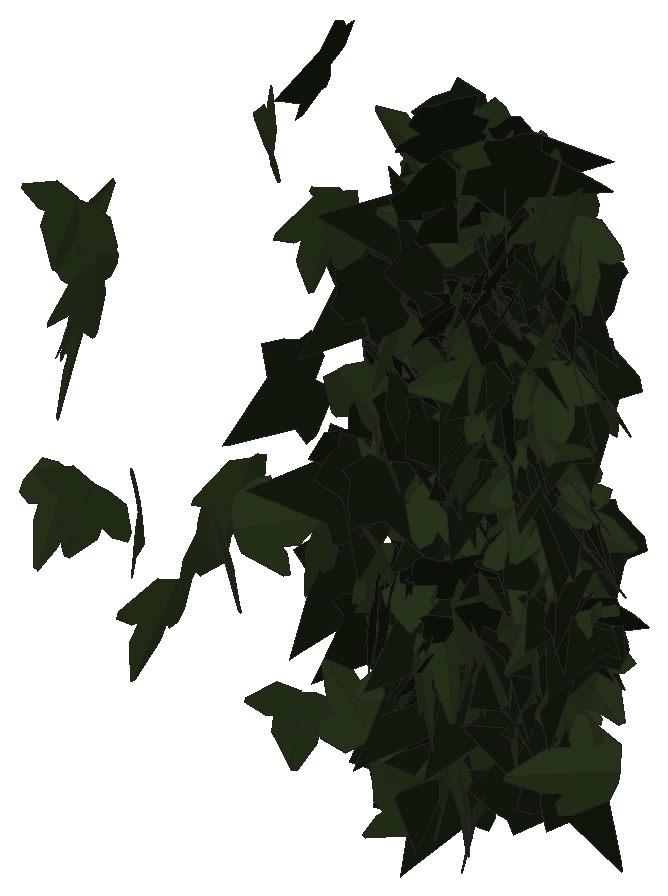
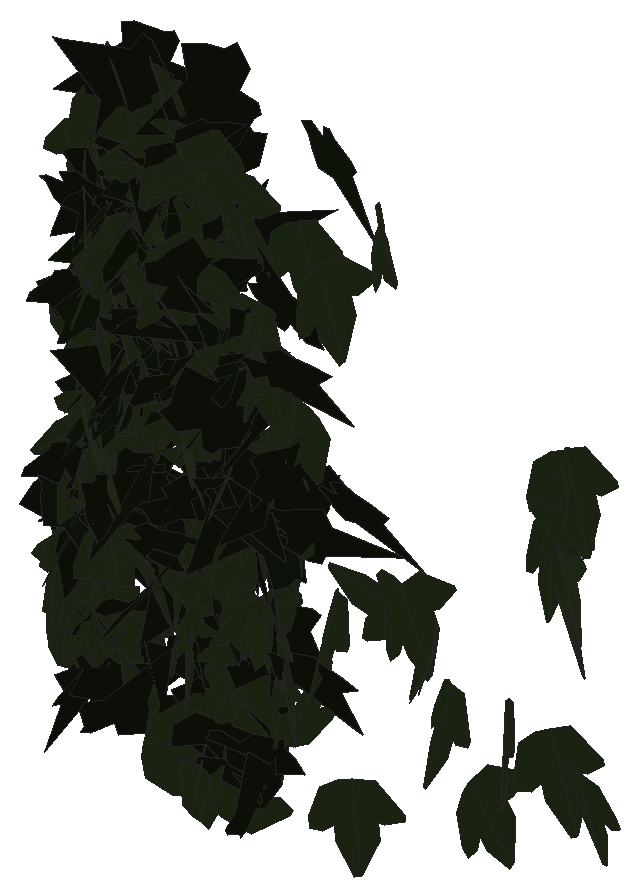
# SketchUp Ruby script. Lengths in inches.
U = 1.inch
M = Sketchup.active_model
def pt(a) = Geom::Point3d.new(a.map { |v| v * U })
def face(e, loops, mat)
  f = e.add_face(loops[0].map { |a| pt(a) })
  loops[1..].each { |l| e.add_face(l.map { |a| pt(a) }).erase! }
  f.material = f.back_material = mat if mat
  f
end
# faces: each face lists its corners as indices into pts; further lists are holes
def faces(e, pts, list, mat = nil) = list.each { |f| face(e, (f[0].is_a?(Array) ? f : [f]).map { |l| l.map { |i| pts[i] } }, mat) }
# xy, xz, yz: faces in a plane at the given z, y or x. An outline is a flat list of corners, or four numbers for a rectangle; further outlines are holes
def ring(l) = l.size == 4 ? [[l[0], l[1]], [l[2], l[1]], [l[2], l[3]], [l[0], l[3]]] : l.each_slice(2).to_a
def flat(e, list, mat, &to3) = list.each { |f| face(e, (f[0].is_a?(Array) ? f : [f]).map { |l| ring(l).map { |u, v| to3.(u, v) } }, mat) }
def xy(e, z, list, mat = nil) = flat(e, list, mat) { |x, y| [x, y, z] }
def xz(e, y, list, mat = nil) = flat(e, list, mat) { |x, z| [x, y, z] }
def yz(e, x, list, mat = nil) = flat(e, list, mat) { |y, z| [x, y, z] }
def lines(e, pts, list) = list.each { |a, b| e.add_line(pt(pts[a]), pt(pts[b])) }
# prism: a flat outline (further loops are holes) pulled along v
def prism(e, loops, v, mat = nil)
  f = face(e, loops, mat); d = Geom::Vector3d.new(v.map { |x| x * U })
  f.pushpull(f.normal.samedirection?(d) ? d.length : -d.length)
end
def box(e, o, s, mat = nil) = prism(e, [[o, [o[0] + s[0], o[1], o[2]], [o[0] + s[0], o[1] + s[1], o[2]], [o[0], o[1] + s[1], o[2]]]], [0, 0, s[2]], mat)
def at(x, y, z, deg = 0) = Geom::Transformation.translation(pt([x, y, z])) * Geom::Transformation.rotation(ORIGIN, Z_AXIS, deg.degrees)
def axes(o, x, y, z) = Geom::Transformation.new([*x, 0, *y, 0, *z, 0, *pt(o).to_a, 1])
def part(name) = M.definitions.add(name)
# library, detail: a bought-in or finely detailed component or shape, given as its bounding box
def library(name, o, s) = part(name).tap { |d| box(d.entities, o, s) }
def detail(e, o, s) = box(e.add_group.entities, o, s)
def put(e, d, t, mat = nil) = e.add_instance(d, t).tap { |i| i.material = mat if mat }
def group(e, t, mat = nil) = e.add_group.tap { |g| g.transformation = t; g.material = mat if mat }.entities
root = M.entities
M.materials.add("efeu1").color = [18, 25, 13]
M.materials.add("efeu2").color = [43, 57, 29]
c1 = part("ivyleaf_9")
p = [[1.54,2.16,1.25],[1.36,2.04,1.19],[-0.21,0.99,0.68],[-0.71,1.11,0.82],[-0.85,0.86,0.67],[-0.8,0.17,0.21],
  [-0.9,-0.01,0.1],[-0.67,-0.16,-0.02],[-0.08,-0.08,-0.05],[-0.03,-0.6,-0.4],[0.65,-0.88,-0.66],[0.83,-0.6,-0.49],
  [1.29,-0.42,-0.43],[1.8125,-0.07,-0.26],[1.21,0.44,0.15]]
faces(c1.entities,p,[[0,1,2,3,4,5,6,7,8,9,10,11,12,13,14]],"efeu1")
c2 = part("ivyleaf_10")
p = [[0,0.5,-0.03],[-0.0625,2.02,-0.43],[-0.19,2.01,-0.46],[-0.54,1.05,-0.29],[-0.52,0.625,-0.18],[-0.83,0.76,-0.28],
  [-1.16,0.64,-0.33],[-1.15,0.33,-0.24],[-0.77,-0.39,0.02],[-0.3,-0.51,0.16],[0.04,-0.48,0.23],[-0.02,2.01,-0.4375],
  [-0.06,2.01,-0.43],[0.04,-0.49,0.23],[0.67,-0.49,0.14],[1.38,0.36,-0.2],[1.375,0.51,-0.24],[0.81,0.65,-0.19],
  [0.62,0.59,-0.15],[0.6,1.09,-0.28],[0.5,1.23,-0.31]]
faces(c2.entities,p,[[0,1,2,3,4,5,6,7,8,9,10],[11,12,0,13,14,15,16,17,18,19,20]],"efeu2")
put(root,c1,axes([6.34,223.31,216.77],[-0.08442,0.02651,-0.44418],[-0.43488,0.14238,0.08583],[0.15641,0.41018,-0.00109]))
put(root,c1,axes([7.9,223.14,221.38],[-0.16025,0.38078,-0.28165],[-0.14438,0.24391,0.4119],[0.45108,0.21335,0.03178]))
put(root,c2,axes([7.45,223.71,219.89],[0.14009,0.04827,-0.42889],[-0.40482,-0.17224,-0.14358],[-0.19289,0.39652,-0.01015]))
put(root,c2,axes([5.9,223.44,217.36],[-0.40342,0.14328,0.1776],[-0.17463,0.05524,-0.41604],[-0.16573,-0.40699,0.00606]))
put(root,c2,axes([8.27,223.6,218.73],[0.38843,0.21317,-0.12492],[-0.11749,-0.05197,-0.43468],[-0.23671,0.37561,0.01075]))
put(root,c1,axes([6.24,223.5,218.32],[-0.00908,-0.31189,-0.31524],[0.03236,0.30203,-0.32408],[0.4686,-0.02691,0.01627]))
put(root,c1,axes([7.67,223.62,220.76],[0.29503,-0.33524,0.04895],[0.08995,0.00794,-0.44395],[0.35437,0.27709,0.07193]))
put(root,c2,axes([4.25,223.52,216.91],[0.16901,-0.0264,-0.42122],[0.43731,-0.01972,0.16404],[-0.03016,-0.43375,0.01818]))
put(root,c1,axes([7.86,223.3,222.82],[0.07338,0.12006,-0.42905],[0.15609,0.38695,0.14187],[0.43699,-0.15838,0.02137]))
put(root,c2,axes([5.65,223.63,214.87],[-0.00989,0.40743,0.15821],[-0.00063,-0.15217,0.42382],[0.4697,0.00837,0.0039]))
put(root,c2,axes([5.68,223.53,221.31],[-0.42118,-0.01919,0.19943],[-0.20608,-0.02225,-0.40589],[0.02919,-0.43401,0.01199]))
put(root,c2,axes([3.75,223.55,216.64],[-0.27006,0.344,-0.0951],[0.06605,-0.06857,-0.44219],[-0.3787,-0.25727,-0.0093]))
put(root,c1,axes([5.87,223.49,220.1875],[-0.29561,0.21016,0.27543],[0.20479,-0.18669,0.35788],[0.3023,0.33197,0.0269]))
put(root,c1,axes([8.32,223.84,218.49],[0.0188,-0.40254,0.17053],[0.05044,-0.16142,-0.41728],[0.46671,0.03366,0.03822]))
put(root,c2,axes([7.61,223.45,220.09],[-0.0146,0.42582,0.09135],[-0.05974,0.08548,-0.43983],[-0.46576,-0.02432,0.05355]))
put(root,c2,axes([7.49,223.74,220.97],[0.17974,-0.44438,0.14221],[0.07423,-0.12322,-0.47886],[0.46064,0.19325,0.02167]))
put(root,c1,axes([7.68,223.9375,220.05],[-0.19316,-0.2849,0.28684],[-0.12506,-0.25185,-0.34865],[0.40959,-0.21126,0.02882]))
put(root,c1,axes([7.85,223.68,221.03],[-0.27086,0.25624,-0.25615],[0.17868,-0.18263,-0.37281],[-0.33974,-0.30035,0.00816]))
put(root,c1,axes([5.77,223.82,218.03],[-0.11443,-0.42164,0.01532],[-0.00533,-0.01395,-0.45214],[0.45562,-0.10606,-0.00144]))
put(root,c1,axes([7.42,223.55,220.71],[0.32523,-0.27615,-0.15525],[-0.10628,0.11339,-0.4246],[0.32194,0.3164,0.01667]))
put(root,c2,axes([7.09,223.78,220.91],[0.19852,-0.34517,0.19814],[0.10232,-0.16538,-0.40666],[0.41332,0.20673,0.00551]))
put(root,c2,axes([7.64,223.53,219.7],[0.11627,0.41869,0.0502],[0.0202,0.04502,-0.44955],[-0.45474,0.10906,-0.00713]))
put(root,c2,axes([8.78,223.91,215.2],[0.01928,0.04885,0.49723],[-0.21576,-0.448,0.05238],[0.45064,-0.21658,0.0038]))
put(root,c2,axes([7.16,223.86,214.02],[0.02072,-0.27912,-0.34642],[0.10789,-0.32166,0.2863],[-0.45677,-0.08864,0.05191]))
put(root,c1,axes([8.18,223.79,219.51],[-0.31383,-0.29925,-0.12837],[0.12827,0.05575,-0.43133],[0.32522,-0.31076,0.04624]))
put(root,c1,axes([7.89,223.42,219.26],[0.04919,-0.08314,0.44153],[-0.11972,0.41039,0.09595],[-0.45162,-0.11785,0.02265]))
put(root,c1,axes([7.43,223.51,219.35],[-0.21801,0.38417,-0.03104],[0.00539,-0.03109,-0.45121],[-0.41612,-0.20167,0.01042]))
put(root,c2,axes([7.89,223.54,218.52],[-0.00122,-0.05645,0.44857],[0.43742,0.15723,0.0225],[-0.1714,0.40164,0.05424]))
put(root,c2,axes([6.75,223.7,216.26],[0.39509,-0.11742,0.21214],[0.22194,-0.02446,-0.39792],[0.12393,0.41814,0.0363]))
put(root,c2,axes([7.98,223.58,218.63],[-0.36368,-0.26549,-0.07601],[0.06353,0.04343,-0.44596],[0.29053,-0.34184,0.00237]))
put(root,c2,axes([6.53,223.61,219.96],[-0.29461,-0.01972,0.3518],[-0.36334,-0.03605,-0.28433],[0.04366,-0.43305,0.00765]))
put(root,c2,axes([7.67,223.64,222.58],[-0.45552,-0.05134,0.09695],[-0.09095,-0.07195,-0.43749],[0.07027,-0.42593,0.06222]))
put(root,c1,axes([8.26,223.7,221.71],[-0.41055,0.07333,0.20628],[-0.20955,0.0413,-0.40262],[-0.09082,-0.42678,-0.00352]))
put(root,c2,axes([7.49,223.81,220.7],[0.08973,-0.46558,0.15868],[0.07998,-0.14534,-0.47168],[0.48534,0.11003,0.04839]))
put(root,c2,axes([8.35,223.66,222.74],[0.284,-0.33926,-0.07337],[-0.04917,0.05397,-0.4464],[0.37099,0.26686,-0.003]))
put(root,c2,axes([8.43,223.64,219.21],[-0.40337,-0.21275,0.06951],[-0.06302,-0.0326,-0.44703],[0.23245,-0.37802,-0.00057]))
put(root,c2,axes([7.34,223.58,218.9],[0.09926,-0.45723,-0.17632],[-0.0433,0.17102,-0.46784],[0.48813,0.10814,-0.00565]))
put(root,c2,axes([3.84,223.82,217.25],[-0.01194,-0.48331,0.12756],[0.03351,-0.12808,-0.48215],[0.49873,-0.00296,0.03545]))
put(root,c1,axes([6.76,223.7,220.89],[-0.18269,-0.37381,0.15028],[0.06298,0.13222,0.42671],[-0.42822,0.17892,-0.00136]))
put(root,c2,axes([7.63,223.71,219.9],[-0.45203,-0.04587,0.11365],[0.11726,0.01243,0.43789],[-0.05133,0.4324,-0.00053]))
put(root,c1,axes([6.43,223.92,221.22],[-0.18491,-0.0378,0.41402],[-0.38126,-0.18915,-0.17658],[0.20288,-0.3899,0.04553]))
put(root,c1,axes([6.79,223.36,222.84],[0.27354,0.20592,0.29903],[0.24286,0.17919,-0.33947],[-0.2948,0.33869,-0.0022]))
put(root,c2,axes([8.15,223.88,220.38],[0.19348,-0.40299,0.22396],[0.12952,-0.1856,-0.44585],[0.44248,0.23054,0.03257]))
put(root,c2,axes([8.32,223.6875,220.06],[0.19006,0.395,-0.04908],[-0.00722,-0.04866,-0.44951],[-0.42958,0.17558,-0.01416]))
put(root,c2,axes([5.09,223.81,221.04],[-0.0852,-0.48239,0.10018],[0.02584,-0.1059,-0.48797],[0.49201,-0.07797,0.04297]))
put(root,c2,axes([7.71,223.57,220.58],[0.04335,-0.00644,-0.45042],[-0.40664,0.2145,-0.03961],[0.23126,0.37838,0.01479]))
put(root,c1,axes([7.47,223.49,221.05],[0.42899,0.17689,0.01302],[0.01072,0.00847,-0.4522],[-0.19122,0.39732,0.00385]))
put(root,c1,axes([6.54,223.89,215.5],[-0.44176,-0.14477,0.03216],[-0.0262,-0.02408,-0.451],[0.15772,-0.4095,0.01515]))
put(root,c1,axes([6.82,223.64,217],[0.36142,0.2653,-0.08609],[0.06706,0.05492,0.44411],[0.29256,-0.34033,0.00456]))
put(root,c2,axes([8.07,223.73,217.875],[0.42982,0.16948,-0.0478],[-0.04605,-0.01719,-0.44987],[-0.18398,0.40026,0.00092]))
put(root,c2,axes([7.22,223.65,222.11],[-0.4457,-0.01243,0.14245],[-0.14773,-0.00784,-0.42937],[0.01541,-0.43475,0.00367]))
put(root,c2,axes([7.5,223.7,221.34],[-0.17632,0.39213,-0.09761],[0.04226,-0.08537,-0.44173],[-0.4334,-0.16785,-0.00336]))
put(root,c2,axes([8.47,223.75,222.28],[-0.11988,-0.48528,0.0114],[-0.00174,-0.01132,-0.49987],[0.48541,-0.11988,0.00103]))
put(root,c2,axes([6.53,223.68,215.79],[-0.1474,0.40916,-0.0587],[0.00871,-0.0568,-0.44845],[-0.44599,-0.13634,0.01064]))
put(root,c2,axes([6.88,223.88,221.36],[0.07607,0.11513,0.43007],[-0.31967,-0.29048,0.13654],[0.33576,-0.30264,0.03256]))
put(root,c2,axes([7.6,223.84,222.28],[-0.13898,0.33603,-0.25421],[0.06725,-0.23741,-0.37351],[-0.44371,-0.14123,0.02301]))
put(root,c2,axes([8.28,223.83,218.73],[0.09753,-0.48386,0.07978],[0.02458,-0.07642,-0.49351],[0.48978,0.10019,0.00888]))
put(root,c1,axes([6.8,223.42,221.76],[0.095,0.03237,0.48982],[0.43016,0.23489,-0.09895],[-0.23652,0.4402,0.01678]))
put(root,c2,axes([7.61,223.6,216.01],[-0.26817,0.20785,-0.30208],[-0.25162,0.17388,0.33654],[0.29238,0.34028,0.01255]))
put(root,c1,axes([7.21,223.89,218.75],[-0.37895,-0.17269,-0.19811],[0.21139,0.02958,-0.40284],[0.18006,-0.39816,0.05599]))
put(root,c2,axes([6.23,223.93,213.8125],[-0.23891,-0.26341,-0.27693],[-0.18593,-0.20315,0.35773],[-0.35926,0.28031,-0.00098]))
put(root,c2,axes([6.03,223.57,218.44],[-0.31407,0.18574,0.27547],[-0.2544,0.12257,-0.35834],[-0.23949,-0.37377,0.01938]))
put(root,c1,axes([5.54,223.86,217.64],[-0.33687,0.02219,0.31449],[-0.32737,-0.03308,-0.32265],[0.00774,-0.43317,0.04075]))
put(root,c2,axes([7.96,223.73,219.55],[-0.28637,0.0566,-0.35378],[-0.36547,0.03989,0.28123],[0.07169,0.42945,0.0205]))
put(root,c1,axes([8.25,223.92,218.86],[0.0765,-0.42865,0.02247],[0.00429,-0.02125,-0.45184],[0.46351,0.07094,0.00048]))
put(root,c1,axes([7.09,223.53,220.67],[-0.03276,0.43341,0.02242],[-0.00664,0.02118,-0.45182],[-0.46861,-0.0306,0.00484]))
put(root,c2,axes([7.11,224.02,215.88],[-0.04675,0.12702,-0.43034],[0.07748,-0.40799,-0.13805],[-0.461,-0.08146,0.02044]))
put(root,c1,axes([5.96,223.89,216.24],[0.03061,0.13804,-0.428],[-0.11768,-0.39695,-0.14627],[-0.45379,0.11225,0.00906]))
put(root,c2,axes([7.25,223.72,222.18],[-0.22063,-0.00476,-0.39938],[0.4138,-0.03225,-0.21156],[-0.02835,-0.43378,0.02011]))
put(root,c2,axes([4.5,223.55,221.78],[-0.0312,0.01566,0.45111],[-0.41305,0.20464,-0.03417],[-0.22166,-0.38354,0.00018]))
put(root,c2,axes([5.95,223.7,217.98],[0.45833,0.08239,-0.05028],[0.05042,0.01318,0.44958],[0.09,-0.42692,0.00418]))
put(root,c1,axes([8.3,224.09,221.27],[-0.01787,-0.09975,0.44001],[0.0125,-0.42334,-0.10333],[0.46929,0.00747,0.01951]))
put(root,c2,axes([8.33,223.87,221.67],[0.20389,-0.38938,0.04614],[0.01773,-0.04134,-0.45003],[0.42288,0.18948,-0.00337]))
put(root,c2,axes([7.6,223.71,220.72],[-0.25982,-0.3433,-0.12081],[0.07304,0.09445,-0.43597],[0.38454,-0.24989,0.00118]))
put(root,c1,axes([7.72,223.42,221.5],[-0.12709,0.28443,-0.31966],[-0.16066,0.27006,0.31914],[0.42279,0.18813,0.02518]))
put(root,c1,axes([7.81,224,220.61],[-0.35008,-0.28308,-0.06591],[0.09155,-0.00155,-0.44372],[0.29962,-0.33028,0.05857]))
put(root,c2,axes([5.47,223.75,219.01],[-0.36215,0.0296,-0.28653],[0.29623,-0.02603,-0.35009],[-0.04254,-0.43321,0.00146]))
put(root,c2,axes([7.52,223.8,222.93],[0.34359,-0.27387,-0.11861],[-0.09012,0.07787,-0.43655],[0.30746,0.32887,0.0046]))
put(root,c2,axes([1.52,223.78,219.82],[-0.44881,-0.08403,0.20374],[-0.19755,-0.0515,-0.45642],[0.09769,-0.49019,0.01303]))
put(root,c1,axes([8.52,224.11,217.09],[-0.21944,-0.36814,0.11588],[0.06317,-0.15412,-0.41866],[0.41057,-0.17304,0.12635]))
put(root,c1,axes([7.7,223.93,221.55],[-0.4629,-0.04246,-0.06338],[0.06467,0.01369,-0.44787],[0.04747,-0.43271,-0.00795]))
put(root,c1,axes([8.18,223.98,216.6875],[-0.27871,-0.14926,-0.32945],[0.36472,-0.00196,-0.28515],[0.10007,-0.40859,0.12172]))
put(root,c1,axes([6.13,223.85,218.84],[0.28368,-0.40562,-0.0707],[-0.02524,0.06856,-0.49463],[0.41096,0.28421,0.01842]))
put(root,c2,axes([7.61,223.65,220.38],[0.15719,0.09602,0.41446],[0.34791,0.23474,-0.18118],[-0.27379,0.35342,0.00773]))
put(root,c1,axes([6.6,223.95,218.85],[0.16588,-0.47138,-0.0168],[-0.00393,0.01643,-0.49971],[0.47166,0.16592,0.00174]))
put(root,c1,axes([8.2,224.14,217.34],[-0.16537,-0.33622,0.23883],[0.02911,-0.25318,-0.36681],[0.43877,-0.10992,0.11435]))
put(root,c1,axes([7.09,223.57,216.68],[0.36854,0.26901,0.02119],[0.01624,0.01382,-0.4519],[-0.29091,0.34157,0.00161]))
put(root,c1,axes([6.9375,224.04,221.32],[0.1541,-0.26078,0.33029],[0.15509,-0.28335,-0.30907],[0.41583,0.20232,-0.00713]))
put(root,c2,axes([1.43,223.93,218.15],[0.31255,-0.38255,0.07725],[0.0486,-0.06005,-0.494],[0.38723,0.31631,-0.00035]))
put(root,c2,axes([8.04,223.79,216.5],[-0.17788,0.39712,-0.06891],[0.02933,-0.06047,-0.44712],[-0.43383,-0.16691,-0.00197]))
put(root,c2,axes([6.77,223.66,218.08],[0.21404,0.31211,0.23837],[0.13334,0.19311,-0.38451],[-0.39638,0.2335,-0.00063]))
put(root,c2,axes([8.26,223.65,219.2],[0.17871,0.34016,0.22338],[0.11234,0.18818,-0.39327],[-0.41971,0.19521,-0.01014]))
put(root,c1,axes([7.65,223.81,222.15],[-0.13413,-0.0405,-0.43152],[-0.41812,-0.14941,0.13568],[-0.16703,0.40653,0.00688]))
put(root,c1,axes([5.92,223.58,216.5],[0.03963,-0.02155,-0.45023],[-0.41039,0.20743,-0.04423],[0.22522,0.38175,-0.00138]))
put(root,c2,axes([2.61,224.02,215.18],[-0.00214,-0.45993,0.19611],[0.01706,-0.19606,-0.45964],[0.4997,0.00472,0.01653]))
put(root,c1,axes([8.25,223.76,218.45],[0.44407,-0.14041,-0.02191],[-0.02094,0.00843,-0.45187],[0.15191,0.41163,0.00178]))
put(root,c1,axes([6.02,223.7,219.51],[0.43056,0.02325,-0.17938],[-0.18567,-0.01445,-0.4153],[-0.02924,0.43414,-0.00422]))
put(root,c1,axes([7.73,223.57,219.72],[0.02311,0.42198,0.10756],[-0.06805,0.10547,-0.43398],[-0.46427,0.00554,0.06896]))
put(root,c2,axes([8.07,224.11,219.76],[0.10338,-0.35687,0.33459],[0.21115,-0.27593,-0.35955],[0.44128,0.21564,0.09366]))
put(root,c2,axes([8.07,224.16,216.81],[-0.01997,-0.18968,0.40667],[0.03098,-0.39106,-0.19587],[0.46835,0.01778,0.0303]))
put(root,c2,axes([6.4,224.1,217.76],[-0.13081,0.19306,0.38534],[0.16589,-0.33818,0.23548],[0.41962,0.19388,0.02703]))
put(root,c1,axes([6.4375,224.06,219.6],[-0.37122,-0.26631,-0.0132],[0.00998,0.00879,-0.45221],[0.28777,-0.34384,-0.00135]))
put(root,c1,axes([7.62,223.68,220.88],[0.34486,0.26544,-0.13482],[-0.10654,-0.08411,-0.43184],[-0.30071,0.33421,-0.00161]))
put(root,c1,axes([6.56,223.84,215.9],[-0.2079,0.35024,-0.17862],[0.07844,-0.156,-0.4155],[-0.41393,-0.20548,0.01097]))
put(root,c2,axes([1.5,223.83,218.67],[0.22504,-0.42546,-0.13542],[-0.06812,0.11716,-0.48128],[0.44127,0.23507,-0.00523]))
put(root,c2,axes([8.45,223.91,221.89],[-0.43326,-0.14968,-0.07976],[0.13025,-0.11775,-0.41706],[0.12661,-0.39109,0.1561]))
put(root,c2,axes([6.14,223.68,219.98],[0.08651,-0.39486,-0.29428],[-0.00707,0.29776,-0.40161],[0.49241,0.07365,0.04593]))
put(root,c2,axes([7.13,223.62,216.76],[-0.16176,0.30998,0.27654],[-0.13697,0.23392,-0.35789],[-0.41927,-0.19601,0.01022]))
put(root,c1,axes([5.11,223.76,222.93],[-0.29403,0.33582,0.05018],[-0.02541,0.04302,-0.44952],[-0.36553,-0.27313,-0.00911]))
put(root,c2,axes([7.375,223.91,216.46],[-0.45498,0.01596,-0.1115],[-0.11561,0.00635,0.43844],[0.0184,0.43466,-0.00231]))
put(root,c1,axes([6.35,223.66,217.32],[-0.09109,0.07229,-0.4374],[-0.44956,0.08052,0.10121],[0.10154,0.42133,0.05571]))
put(root,c2,axes([8.37,223.9,217.38],[0.4454,0.12427,0.06328],[0.06091,0.0237,-0.4479],[-0.13646,0.4162,0.00661]))
put(root,c1,axes([7.7,223.67,222.2],[0.12681,0.41825,-0.02331],[-0.01703,-0.01885,-0.45168],[-0.45204,0.11805,0.01047]))
put(root,c2,axes([7.02,224.13,222.29],[0.00604,-0.08871,-0.44286],[0.25334,-0.35801,0.08077],[-0.3956,-0.23062,0.04496]))
put(root,c1,axes([7.9375,224.12,221.45],[0.1818,-0.43963,0.15387],[0.05122,-0.14531,-0.47567],[0.46295,0.18872,-0.0078]))
put(root,c2,axes([7.03,224.01,219.64],[-0.26878,0.23302,-0.28097],[0.15053,-0.23972,-0.34857],[-0.35469,-0.27832,0.06498]))
put(root,c1,axes([7.53,223.875,218.83],[-0.12018,0.04887,-0.43439],[-0.41331,-0.19086,0.08281],[-0.18826,0.38783,0.09549]))
put(root,c2,axes([7.33,223.8,216.92],[-0.35212,0.05941,0.29305],[-0.2993,0.05095,-0.34466],[-0.08452,-0.4279,-0.00035]))
put(root,c1,axes([6.61,223.66,220.3],[0.39916,0.09792,0.28475],[0.27364,0.07937,-0.41088],[-0.12567,0.48385,0.00977]))
put(root,c1,axes([8.09,223.97,217.8125],[0.02583,-0.40556,-0.16171],[-0.01826,0.15474,-0.42244],[0.46873,0.02838,-0.00755]))
put(root,c2,axes([6.15,223.99,215.34],[0.39765,0.24072,-0.1842],[-0.15715,-0.09609,-0.46483],[-0.25919,0.42757,-0.00076]))
put(root,c1,axes([7.7,223.85,222.71],[0.3236,0.12731,-0.30005],[0.26169,0.16177,0.33595],[0.21798,-0.38321,0.04213]))
put(root,c1,axes([7.13,224.1,215.65],[-0.4146,-0.20295,-0.02684],[0.02885,0.00469,-0.45152],[0.21906,-0.38473,0.00866]))
put(root,c1,axes([8.32,224.11,217.91],[-0.31247,-0.16005,-0.29398],[0.33444,-0.02155,-0.31693],[0.10597,-0.40391,0.1334]))
put(root,c2,axes([1.66,223.87,219],[-0.01494,-0.48235,-0.13084],[0.01399,0.13044,-0.48248],[0.49958,-0.01808,0.0096]))
put(root,c1,axes([6.74,224.25,218.1875],[0.22673,-0.243,-0.30517],[0.21462,-0.216,0.3339],[-0.35106,-0.28899,0.00704]))
put(root,c2,axes([6.58,223.87,216.54],[0.20642,0.45354,0.04116],[-0.03079,-0.03119,0.49808],[0.45436,-0.20816,0.01505]))
put(root,c2,axes([7.37,224.09,218.7],[0.17212,-0.21417,0.35719],[0.35989,-0.14008,-0.25166],[0.24812,0.35176,0.11725]))
put(root,c1,axes([5.82,223.63,217.39],[-0.13806,0.39143,-0.14584],[-0.04879,0.13276,0.42825],[0.4464,0.13557,0.0017]))
put(root,c1,axes([6.48,224.21,216.26],[-0.4072,-0.20129,0.08416],[-0.02509,-0.12387,-0.433],[0.23296,-0.36519,0.10048]))
put(root,c1,axes([6.43,224.04,216.43],[-0.35183,0.18066,-0.23363],[0.20774,-0.11627,-0.38733],[-0.23189,-0.37825,0.00748]))
put(root,c2,axes([1.6,223.95,216.15],[-0.44356,-0.08668,0.21387],[-0.2043,-0.06798,-0.45127],[0.10731,-0.48771,0.02489]))
put(root,c1,axes([8.04,223.9,221.49],[-0.11767,-0.11592,-0.47193],[0.34461,0.32245,-0.16513],[0.34263,-0.36413,0.00401]))
put(root,c1,axes([6.14,224.06,214.69],[-0.27419,-0.28253,-0.22049],[0.15133,0.15911,-0.39503],[0.35019,-0.28998,-0.00193]))
put(root,c2,axes([6.53,224.07,221.625],[0.31468,0.14888,-0.29811],[-0.28585,-0.11121,-0.33988],[-0.19994,0.39331,0.01673]))
put(root,c2,axes([7.49,223.73,222.28],[-0.14134,-0.19163,-0.38265],[0.23678,0.29558,-0.2412],[0.38035,-0.25522,0.00796]))
put(root,c2,axes([7.41,224.1,216.52],[0.32968,-0.23106,0.21478],[0.19912,-0.0976,-0.39698],[0.26902,0.3554,0.03062]))
put(root,c2,axes([5.94,223.94,219.76],[-0.38339,-0.05491,0.25516],[-0.26339,-0.02795,-0.37349],[0.06598,-0.43061,-0.00829]))
put(root,c2,axes([7.77,224.11,222.13],[0.10333,0.19486,0.39204],[-0.30636,-0.25803,0.21359],[0.34085,-0.29099,0.07313]))
put(root,c1,axes([8,223.86,217.9375],[-0.07999,-0.13863,-0.42184],[0.19693,0.36233,-0.16342],[0.41896,-0.19678,-0.00372]))
put(root,c1,axes([8.1,223.82,219.19],[0.3075,-0.17622,-0.28878],[-0.20676,0.20981,-0.34265],[0.28879,0.33786,0.06217]))
put(root,c2,axes([7.56,223.72,219.94],[0.16965,0.13235,0.39879],[0.19087,0.34779,-0.20014],[-0.39434,0.22528,0.07469]))
put(root,c2,axes([8.35,223.92,217.68],[-0.46402,0.05066,0.0472],[-0.04885,0.00397,-0.44993],[-0.05486,-0.43202,0.00141]))
put(root,c2,axes([6.45,223.76,219.72],[0.07009,0.06117,-0.49127],[-0.36737,0.33903,-0.0102],[0.33186,0.36238,0.09247]))
put(root,c1,axes([7.92,223.93,221.3],[-0.06287,-0.31796,-0.38072],[0.11439,0.36412,-0.323],[0.48266,-0.12772,0.02696]))
put(root,c1,axes([6.51,223.96,215.17],[0.06539,0.33569,-0.28075],[-0.08935,-0.25846,-0.35356],[-0.45657,0.09866,0.02899]))
put(root,c2,axes([8.18,224.01,217.61],[-0.3027,0.00039,0.34598],[-0.34926,-0.10235,-0.28323],[0.08427,-0.42279,0.06888]))
put(root,c2,axes([6.5625,224.04,214.54],[-0.31716,0.23274,-0.22978],[0.16615,-0.16073,-0.38875],[-0.30416,-0.33049,0.02724]))
put(root,c2,axes([6.38,223.97,217.36],[-0.47108,-0.13338,0.10145],[-0.0972,-0.02912,-0.4896],[0.13651,-0.481,0.0015]))
put(root,c2,axes([6.4,223.96,221.9],[-0.42249,0.07242,-0.18296],[0.1862,-0.03512,-0.41374],[-0.08687,-0.42749,0.003]))
put(root,c2,axes([5.76,224.1,216.47],[0.0639,-0.42509,0.07374],[0.00089,-0.07145,-0.44625],[0.46543,0.05849,-0.00927]))
put(root,c2,axes([4.53,224.01,214.51],[-0.4247,-0.17009,0.07822],[-0.06292,-0.0544,-0.44474],[0.19074,-0.39665,0.02746]))
put(root,c2,axes([8.55,223.84,221.35],[0.13479,-0.37384,-0.30344],[-0.07833,0.29389,-0.39686],[0.47508,0.15452,0.02066]))
put(root,c1,axes([8.41,223.86,217.17],[0.2522,-0.21603,-0.30856],[-0.20044,0.23387,-0.32902],[0.34195,0.29641,0.03471]))
put(root,c1,axes([7.71,224.14,218.74],[0.271,-0.3253,0.14869],[0.10443,-0.10591,-0.42711],[0.36928,0.26868,0.01167]))
put(root,c2,axes([1.53,223.71,219.3],[0.08767,-0.25573,0.42061],[-0.15946,0.38944,0.27002],[-0.46571,-0.18149,-0.01327]))
put(root,c1,axes([6.64,224.2,214.28],[-0.41872,-0.18796,-0.06226],[0.06561,0.01183,-0.4478],[0.20269,-0.39212,0.01634]))
put(root,c2,axes([6.93,224.17,220.94],[-0.34788,-0.23217,0.274],[-0.1656,-0.2348,-0.4092],[0.31867,-0.37546,0.08647]))
put(root,c2,axes([8.31,224.01,215.69],[-0.37569,0.17319,-0.20333],[0.19154,-0.08242,-0.4041],[-0.20708,-0.39043,-0.00489]))
put(root,c2,axes([6.77,224.01,214.4],[-0.28361,0.34002,-0.07091],[-0.0006,-0.08594,-0.44348],[-0.37453,-0.25734,0.0544]))
put(root,c1,axes([8.52,224.2,216.92],[-0.42701,-0.12817,-0.13347],[0.14455,0.00154,-0.43045],[0.13219,-0.41569,0.03955]))
put(root,c1,axes([5.46,223.75,218.42],[0.00912,-0.03648,-0.45072],[-0.02746,0.43268,-0.0384],[0.46891,0.02605,0.00652]))
put(root,c1,axes([7.2,224.21,219.33],[-0.33104,-0.29947,-0.07774],[0.049,0.06049,-0.44551],[0.32973,-0.30965,-0.01185]))
put(root,c1,axes([7.4,224.22,217.03],[-0.43901,-0.07279,0.14218],[-0.14026,-0.04901,-0.42875],[0.09114,-0.42606,0.02503]))
put(root,c1,axes([4.5625,224.14,218.5625],[-0.46608,0.03834,0.04052],[-0.04176,0.0051,-0.45058],[-0.04174,-0.43328,-0.00172]))
put(root,c1,axes([7.83,224.18,217.7],[-0.1999,-0.36777,-0.14602],[0.08457,0.11765,-0.42786],[0.41665,-0.20032,0.01679]))
put(root,c1,axes([7.23,224.18,220.5625],[-0.44951,-0.05832,-0.11669],[0.12147,0.00566,-0.43698],[0.06241,-0.43104,0.01005]))
put(root,c1,axes([8.34,224.15,220.14],[-0.17494,-0.40724,-0.23141],[0.0984,0.20956,-0.44317],[0.45795,-0.20059,0.00682]))
put(root,c2,axes([6.09,224.02,218.48],[-0.40439,0.01148,-0.22995],[0.2371,-0.03704,-0.38865],[-0.03098,-0.43327,0.02713]))
put(root,c1,axes([6.875,224.32,222.5625],[-0.26724,-0.34631,0.09341],[-0.0579,-0.07208,-0.44265],[0.38203,-0.25318,-0.00174]))
put(root,c2,axes([6.12,224.375,217.22],[-0.01691,-0.02124,0.45157],[0.17474,-0.40355,-0.01446],[0.43577,0.161,0.02332]))
put(root,c2,axes([8.24,224.28,217.09],[0.01577,-0.14284,-0.42705],[0.28798,-0.32156,0.12619],[-0.37085,-0.25577,0.07983]))
put(root,c1,axes([8.52,223.88,217.18],[0.30932,0.30249,-0.13031],[-0.099,-0.08573,-0.43316],[-0.33946,0.30063,0.00759]))
put(root,c2,axes([6.43,224.06,219.77],[0.17033,0.40328,-0.04313],[-0.00893,-0.04129,-0.45028],[-0.43774,0.15776,-0.0076]))
put(root,c2,axes([7.64,224.12,220.09],[0.4327,-0.05746,0.16576],[0.17217,-0.01066,-0.42078],[0.06194,0.43106,0.01169]))
put(root,c2,axes([6.51,224.32,213.93],[0.00925,-0.31186,-0.31527],[0.00203,-0.30317,0.32442],[-0.4697,-0.00745,-0.00481]))
put(root,c2,axes([6.3,223.83,215.33],[0.09889,-0.26561,0.34539],[-0.1069,0.31707,0.29212],[-0.44666,-0.13469,0.00655]))
put(root,c2,axes([0.99,224.125,215.95],[0.45538,-0.20484,-0.02595],[-0.02216,0.01399,-0.49931],[0.20528,0.4559,0.00366]))
put(root,c2,axes([5.78,224.1,216.66],[0.16929,0.45974,-0.0999],[-0.03495,-0.09358,-0.48992],[-0.46917,0.17286,0.00045]))
put(root,c2,axes([2.3,223.88,216.25],[0.23941,-0.31149,-0.30928],[-0.07,0.32069,-0.37717],[0.43334,0.2239,0.10994]))
put(root,c1,axes([7.8,224.22,218.88],[0.29002,-0.31921,0.25297],[0.18481,-0.1736,-0.43094],[0.36295,0.34346,0.0173]))
put(root,c2,axes([8.29,224.1,218.36],[0.1018,0.05402,-0.43806],[-0.45863,0.01396,-0.09697],[0.00209,0.43141,0.05799]))
put(root,c2,axes([7.81,223.88,219.05],[-0.00097,-0.32031,-0.30609],[0.0158,0.29413,-0.33296],[0.46953,-0.01056,0.01058]))
put(root,c2,axes([8.0625,224.3,217.6875],[-0.06372,-0.0804,0.44035],[-0.28566,-0.33066,-0.10363],[0.36749,-0.27097,-0.0042]))
put(root,c1,axes([7.78,224.27,217.76],[0.00752,0.10546,-0.43884],[-0.07484,-0.41636,-0.10941],[-0.46374,0.0689,0.01054]))
put(root,c1,axes([6.9,224.37,219.49],[-0.23576,-0.4389,0.04229],[-0.01495,-0.03997,-0.49818],[0.44067,-0.23616,0.00573]))
put(root,c2,axes([7.91,224.32,220.8],[0.07394,0.21253,-0.38826],[-0.24298,-0.30431,-0.22307],[-0.39523,0.22684,0.06451]))
put(root,c1,axes([6.86,224.42,217.88],[-0.36962,-0.28385,0.18114],[-0.12692,-0.13169,-0.46535],[0.31189,-0.38998,0.0253]))
put(root,c1,axes([8.18,223.89,215.17],[-0.41886,0.19512,-0.02824],[-0.02818,0.00855,0.4515],[0.21088,0.38869,0.00424]))
put(root,c1,axes([7.72,224.46,218.99],[-0.17219,-0.19144,0.37086],[-0.16238,-0.32782,-0.25294],[0.40583,-0.21239,0.05614]))
put(root,c2,axes([7.53,223.82,221.8],[0.04043,-0.17929,0.41034],[0.03694,0.39602,0.18377],[-0.4666,0.01581,0.05011]))
put(root,c2,axes([8.59,223.97,216.49],[-0.14677,-0.42457,-0.21954],[0.06529,0.20969,-0.44918],[0.47349,-0.16052,-0.00612]))
put(root,c2,axes([8.45,224.19,217.39],[-0.01533,-0.43078,0.06108],[0.0318,-0.05958,-0.44709],[0.46847,-0.01005,0.03234]))
put(root,c2,axes([7.18,224.39,215.15],[-0.03764,0.05097,-0.49597],[0.24911,-0.42893,-0.06299],[-0.43189,-0.25184,0.0069]))
put(root,c2,axes([8.23,224.06,217.67],[0.02733,-0.4795,-0.13903],[-0.02471,0.13777,-0.48001],[0.49864,0.03311,-0.01617]))
put(root,c2,axes([6.53,224.31,216.52],[0.04156,0.30117,-0.32397],[-0.08174,-0.30326,-0.31465],[-0.46076,0.08097,0.0266]))
put(root,c2,axes([8.26,223.96,218.27],[-0.2182,-0.12538,-0.37883],[0.35539,0.15771,-0.24627],[0.21634,-0.38553,0.02247]))
put(root,c1,axes([7.8,224.3,219.84],[-0.42896,-0.1774,0.00157],[-0.00135,-0.00091,-0.4524],[0.19159,-0.39718,0.00033]))
put(root,c1,axes([7.66,224.21,216.09],[-0.06522,-0.4542,-0.19862],[0.02971,0.19639,-0.45885],[0.49484,-0.07166,0.00137]))
put(root,c2,axes([8.17,224.36,215.43],[-0.07197,0.2307,0.37722],[0.11285,-0.34735,0.24972],[0.45033,0.12391,-0.00229]))
put(root,c2,axes([7.99,224.26,220.68],[0.24963,0.13289,-0.35746],[-0.32239,-0.17039,-0.27728],[-0.23337,0.37753,0.00068]))
put(root,c1,axes([6.03,223.82,217.96],[0.32007,0.29153,0.13321],[0.08897,0.09882,-0.43216],[-0.33219,0.30736,0.0126]))
put(root,c1,axes([6.66,223.95,217.73],[-0.0338,0.02441,0.45051],[-0.27663,0.34951,-0.03973],[-0.37821,-0.25782,-0.0112]))
put(root,c2,axes([6.24,224.03,222],[0.14085,-0.01579,0.43128],[-0.44533,0.04409,0.13661],[-0.05055,-0.43247,-0.00182]))
put(root,c2,axes([8.43,224.0625,216.45],[-0.38513,-0.15911,-0.19936],[0.20871,0.03456,-0.40371],[0.16979,-0.40338,0.04404]))
put(root,c1,axes([5.5,224.3,220.07],[-0.45379,-0.10166,0.05038],[-0.0504,-0.01314,-0.44958],[0.11068,-0.42275,0.00186]))
put(root,c1,axes([6.36,224.125,218.36],[0.08545,0.1118,-0.42939],[-0.36296,-0.24349,-0.13555],[-0.28578,0.34269,0.04378]))
put(root,c1,axes([7.43,224.37,216.3],[0.04689,-0.41897,0.113],[0.01415,-0.10788,-0.43806],[0.46724,0.04531,0.00192]))
put(root,c2,axes([7.77,224.09,220.39],[0.32319,-0.22476,-0.23058],[-0.19236,0.13205,-0.38922],[0.28154,0.34824,-0.00124]))
put(root,c2,axes([7.88,224.13,218.0625],[-0.24593,-0.37047,-0.01157],[0.01246,0.00597,-0.4522],[0.4001,-0.2279,0.00697]))
put(root,c1,axes([7.77,224.14,221.03],[0.40027,-0.20335,0.10664],[0.095,-0.05284,-0.43963],[0.22687,0.3809,-0.00405]))
put(root,c2,axes([8.54,224.18,219.57],[-0.46134,0.08216,0.0019],[-0.00137,-0.01625,0.45208],[0.08874,0.42686,0.01684]))
put(root,c1,axes([6.5,224,219.78],[0.4682,-0.018,-0.0323],[-0.03261,0.02065,-0.4508],[0.02096,0.43414,0.0201]))
put(root,c1,axes([8.12,224.28,214.74],[-0.0782,0.01686,0.44574],[-0.46024,-0.0523,-0.07273],[0.05272,-0.43152,0.02623]))
put(root,c2,axes([6.76,224.22,218.58],[0.1841,-0.39873,0.03576],[0.0172,-0.03058,-0.45098],[0.43188,0.17118,0.00272]))
put(root,c1,axes([7.21,223.91,219.87],[-0.13563,0.26139,0.3372],[-0.20973,0.26284,-0.29859],[-0.39791,-0.22764,0.04244]))
put(root,c2,axes([3.16,223.91,216.2],[0.05828,-0.347,-0.35524],[0.00094,0.35775,-0.3493],[0.49659,0.04005,0.04235]))
put(root,c1,axes([7.73,224.05,221.23],[0.28639,-0.25638,-0.23982],[-0.15598,0.18158,-0.38268],[0.33818,0.30087,0.02659]))
put(root,c1,axes([7.71,224.03,217.86],[0.41286,-0.06753,-0.20414],[-0.20794,0.03841,-0.4037],[0.0838,0.42801,0.00402]))
put(root,c2,axes([8.4,224.1,220.04],[-0.23255,0.37647,-0.03494],[0.01734,-0.02952,-0.45105],[-0.40784,-0.21592,0.00075]))
put(root,c1,axes([8.49,224.3,221.41],[-0.46578,-0.05463,0.01604],[-0.0165,-0.0021,-0.45212],[0.05904,-0.43155,0.00017]))
put(root,c1,axes([8.26,224.11,214.96],[0.16245,-0.32861,-0.2518],[-0.09727,0.22495,-0.37572],[0.42995,0.17505,0.01013]))
put(root,c2,axes([7.91,224.44,216],[-0.0333,0.17678,-0.41211],[-0.10073,-0.39067,-0.17372],[-0.45767,0.07312,0.06822]))
put(root,c2,axes([4.82,223.9375,216.85],[0.13842,-0.34166,-0.3378],[0.02053,0.35543,-0.35107],[0.48002,0.08332,0.11242]))
put(root,c1,axes([8.03,224.3,218.71],[0.28493,-0.40547,0.06639],[0.0327,-0.05816,-0.49553],[0.40957,0.28672,-0.00662]))
put(root,c1,axes([7.92,223.89,218.83],[0.03849,-0.02324,0.45023],[0.3277,0.31159,-0.00858],[-0.33443,0.30264,0.04341]))
put(root,c2,axes([6.95,224.33,220.64],[0.18959,0.29845,-0.27385],[-0.17588,-0.20874,-0.35896],[-0.39222,0.23787,0.02859]))
put(root,c2,axes([6.51,224.2,222.17],[0.41442,-0.1133,-0.17754],[-0.17765,0.04572,-0.4161],[0.13193,0.41749,-0.00262]))
put(root,c2,axes([7.69,224.23,219.59],[0.36103,-0.27718,-0.02645],[-0.02059,0.01684,-0.45163],[0.2999,0.33483,0.00082]))
put(root,c1,axes([6.86,224.42,220.7],[-0.16778,-0.06164,0.41767],[-0.40361,-0.14707,-0.17382],[0.17222,-0.40472,-0.00045]))
put(root,c2,axes([8.29,224.125,216.75],[0.07334,0.07474,0.44004],[-0.46385,-0.00028,0.07174],[0.0131,-0.42853,0.07671]))
put(root,c1,axes([8.02,224.35,220.15],[0.26431,-0.34604,0.24576],[0.19152,-0.16112,-0.43285],[0.37876,0.32295,0.04738]))
put(root,c2,axes([7.625,223.97,220.86],[-0.1103,-0.13748,-0.41586],[0.32882,0.26155,-0.17439],[0.3169,-0.31924,0.03621]))
put(root,c1,axes([6.41,224.39,219],[0.08379,0.01816,0.44475],[-0.44322,-0.12031,0.08275],[0.13132,-0.41764,-0.00449]))
put(root,c1,axes([5.93,224.03,213.94],[-0.11645,-0.21753,0.37538],[0.16309,0.32788,0.25243],[-0.42492,0.18546,-0.00599]))
put(root,c2,axes([6.89,224.26,220.97],[0.24704,0.00331,-0.38479],[-0.39955,-0.00527,-0.23791],[-0.00672,0.43496,0.00004]))
put(root,c1,axes([7.82,224.23,214.51],[-0.33112,-0.3619,0.09692],[0.07704,0.06081,0.49027],[-0.36664,0.33961,0.01549]))
put(root,c2,axes([8.1,224.38,218.51],[0.25323,-0.3999,0.16111],[0.0811,-0.13933,-0.4733],[0.42343,0.26584,-0.0057]))
put(root,c2,axes([7,224.14,222.42],[-0.3974,-0.1665,-0.16802],[0.16385,0.05649,-0.4199],[0.18957,-0.39788,0.0107]))
put(root,c2,axes([7.9375,224.2,216.78],[-0.22235,-0.38134,-0.03921],[0.0249,0.0304,-0.45066],[0.4131,-0.20708,0.00606]))
put(root,c2,axes([7.9375,224.18,217.59],[0.34176,-0.29475,0.04886],[-0.02577,0.04327,0.44947],[-0.32132,-0.31698,0.01593]))
put(root,c2,axes([6.84,224.57,214.66],[-0.02992,-0.11843,0.48485],[-0.10954,-0.47232,-0.12213],[0.48694,-0.11353,0.00232]))
put(root,c2,axes([7.9,224.46,215.88],[0.12971,0.0988,-0.4225],[-0.31733,-0.28075,-0.16135],[-0.32123,0.31724,-0.01121]))
put(root,c1,axes([5.04,224.39,216.28],[-0.45359,-0.10157,-0.05218],[0.05276,0.01145,-0.44938],[0.11039,-0.42282,0.00037]))
put(root,c2,axes([5.375,224.2,216.17],[0.29448,-0.38291,-0.1291],[-0.04489,0.12775,-0.48131],[0.40158,0.29506,0.04086]))
put(root,c2,axes([6.87,224.07,216.07],[0.20695,-0.34769,-0.29374],[-0.06984,0.2946,-0.39791],[0.44977,0.20573,0.07337]))
put(root,c1,axes([8.28,224.32,217.97],[-0.11845,-0.4255,-0.23435],[0.05563,0.22775,-0.44163],[0.48257,-0.1307,-0.00661]))
put(root,c2,axes([6.53,224.03,222.36],[0.16315,0.176,0.38273],[0.23737,0.29549,-0.24079],[-0.37115,0.26634,0.01424]))
put(root,c2,axes([5.95,224.05,216.16],[0.24623,0.39272,-0.18746],[0.08909,0.16533,0.46339],[0.42595,-0.2616,0.01144]))
put(root,c1,axes([8.61,224.17,217.35],[-0.19419,0.38721,-0.08678],[0.03897,-0.07525,-0.444],[-0.42601,-0.18339,-0.00106]))
put(root,c2,axes([7.82,224.28,215.73],[0.40823,0.20847,-0.05587],[-0.0569,-0.01567,-0.44877],[-0.22544,0.38147,0.0121]))
put(root,c2,axes([6.85,224.34,218.95],[0.43292,0.06151,-0.24249],[-0.23711,-0.05363,-0.43692],[-0.07976,0.4933,-0.01726]))
